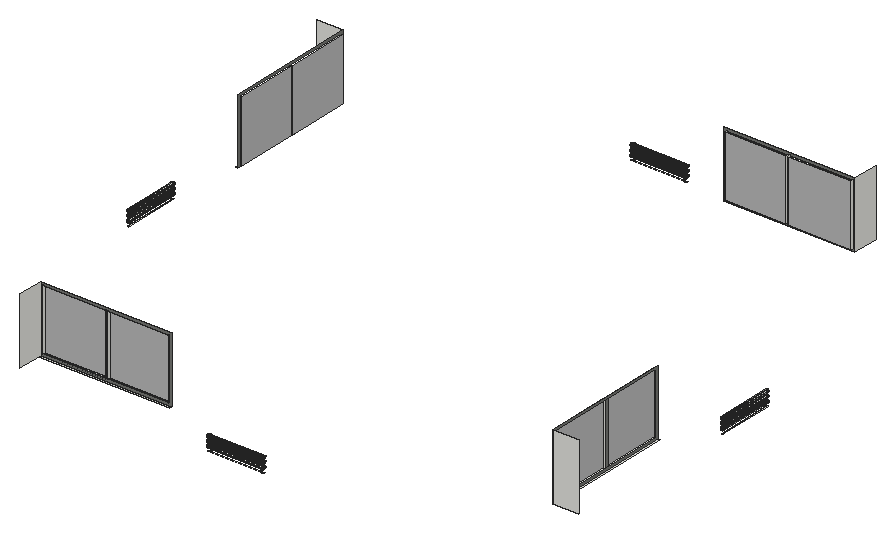
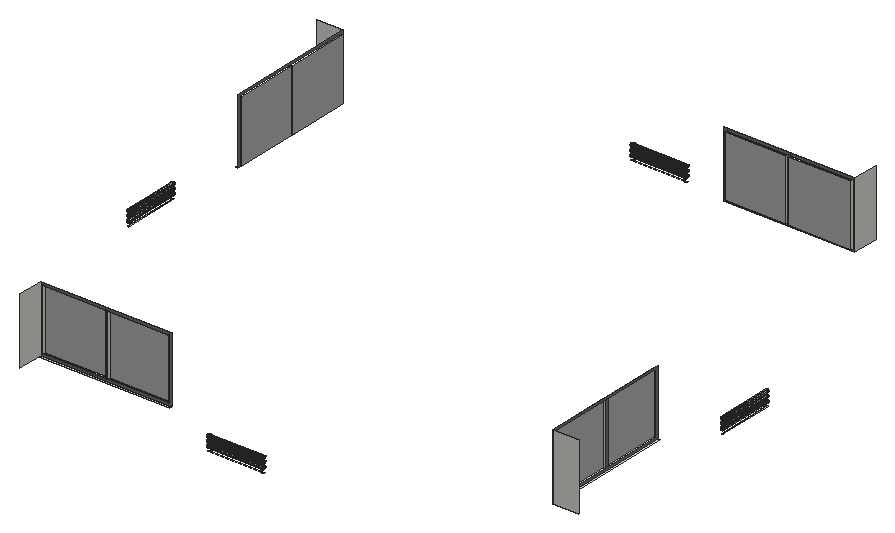
# SketchUp Ruby script. Lengths in inches.
U = 1.inch
M = Sketchup.active_model
def pt(a) = Geom::Point3d.new(a.map { |v| v * U })
def face(e, loops, mat)
  f = e.add_face(loops[0].map { |a| pt(a) })
  loops[1..].each { |l| e.add_face(l.map { |a| pt(a) }).erase! }
  f.material = f.back_material = mat if mat
  f
end
# faces: each face lists its corners as indices into pts; further lists are holes
def faces(e, pts, list, mat = nil) = list.each { |f| face(e, (f[0].is_a?(Array) ? f : [f]).map { |l| l.map { |i| pts[i] } }, mat) }
# xy, xz, yz: faces in a plane at the given z, y or x. An outline is a flat list of corners, or four numbers for a rectangle; further outlines are holes
def ring(l) = l.size == 4 ? [[l[0], l[1]], [l[2], l[1]], [l[2], l[3]], [l[0], l[3]]] : l.each_slice(2).to_a
def flat(e, list, mat, &to3) = list.each { |f| face(e, (f[0].is_a?(Array) ? f : [f]).map { |l| ring(l).map { |u, v| to3.(u, v) } }, mat) }
def xy(e, z, list, mat = nil) = flat(e, list, mat) { |x, y| [x, y, z] }
def xz(e, y, list, mat = nil) = flat(e, list, mat) { |x, z| [x, y, z] }
def yz(e, x, list, mat = nil) = flat(e, list, mat) { |y, z| [x, y, z] }
def lines(e, pts, list) = list.each { |a, b| e.add_line(pt(pts[a]), pt(pts[b])) }
# prism: a flat outline (further loops are holes) pulled along v
def prism(e, loops, v, mat = nil)
  f = face(e, loops, mat); d = Geom::Vector3d.new(v.map { |x| x * U })
  f.pushpull(f.normal.samedirection?(d) ? d.length : -d.length)
end
def box(e, o, s, mat = nil) = prism(e, [[o, [o[0] + s[0], o[1], o[2]], [o[0] + s[0], o[1] + s[1], o[2]], [o[0], o[1] + s[1], o[2]]]], [0, 0, s[2]], mat)
def at(x, y, z, deg = 0) = Geom::Transformation.translation(pt([x, y, z])) * Geom::Transformation.rotation(ORIGIN, Z_AXIS, deg.degrees)
def axes(o, x, y, z) = Geom::Transformation.new([*x, 0, *y, 0, *z, 0, *pt(o).to_a, 1])
def part(name) = M.definitions.add(name)
# library, detail: a bought-in or finely detailed component or shape, given as its bounding box
def library(name, o, s) = part(name).tap { |d| box(d.entities, o, s) }
def detail(e, o, s) = box(e.add_group.entities, o, s)
def put(e, d, t, mat = nil) = e.add_instance(d, t).tap { |i| i.material = mat if mat }
def group(e, t, mat = nil) = e.add_group.tap { |g| g.transformation = t; g.material = mat if mat }.entities
root = M.entities
M.materials.add("[Metal Seamed]").color = [118, 119, 115]
M.materials.add("[Mirror 01]").color = [185, 185, 185]
xy(root,1253.76,[[306.65,96.8125,641.22,102.8125],[1482,271.47,1488,606.03],[132,943.59,138,1278.16],[978.78,1446.8125,1313.35,1452.8125]])
xy(root,1259.76,[[312.65,102.8125,473.9375,108.8125],[479.9375,102.8125,635.22,108.8125],[1476,277.47,1482,438.75],[1476,444.75,1482,600.03],[138,949.59,144,1104.875],
  [138,1110.875,144,1272.16],[984.78,1440.8125,1140.0625,1446.8125],[1146.0625,1440.8125,1307.35,1446.8125]])
xz(root,102.8125,[[[306.65,1253.76,641.22,1422.625],[312.65,1259.76,635.22,1416.625]],[473.9375,1259.76,479.9375,1416.625]],"[Metal Seamed]")
xz(root,108.8125,[[312.65,1259.76,473.9375,1416.625],[479.9375,1259.76,635.22,1416.625]],"[Mirror 01]")
xz(root,271.47,[[1482,1253.76,1548,1422.625]])
xz(root,277.47,[[1476,1259.76,1482,1416.625]])
xz(root,438.75,[[1476,1259.76,1482,1416.625]])
xz(root,444.75,[[1476,1259.76,1482,1416.625]])
xz(root,600.03,[[1476,1259.76,1482,1416.625]])
xz(root,949.59,[[138,1259.76,144,1416.625]])
xz(root,1104.875,[[138,1259.76,144,1416.625]])
xz(root,1110.875,[[138,1259.76,144,1416.625]])
xz(root,1272.16,[[138,1259.76,144,1416.625]])
xz(root,1278.16,[[72,1253.76,138,1422.625]])
xz(root,1440.8125,[[984.78,1259.76,1140.0625,1416.625],[1146.0625,1259.76,1307.35,1416.625]],"[Mirror 01]")
xz(root,1446.8125,[[[978.78,1253.76,1313.35,1422.625],[984.78,1259.76,1307.35,1416.625]],[1140.0625,1259.76,1146.0625,1416.625]],"[Metal Seamed]")
yz(root,138,[[[943.59,1253.76,1278.16,1422.625],[949.59,1259.76,1272.16,1416.625]],[1104.875,1259.76,1110.875,1416.625]],"[Metal Seamed]")
yz(root,144,[[949.59,1259.76,1104.875,1416.625],[1110.875,1259.76,1272.16,1416.625]],"[Mirror 01]")
yz(root,306.65,[[36.8125,1253.76,102.8125,1422.625]])
yz(root,312.65,[[102.8125,1259.76,108.8125,1416.625]])
yz(root,473.9375,[[102.8125,1259.76,108.8125,1416.625]],"[Metal Seamed]")
yz(root,479.9375,[[102.8125,1259.76,108.8125,1416.625]])
yz(root,635.22,[[102.8125,1259.76,108.8125,1416.625]],"[Metal Seamed]")
yz(root,984.78,[[1440.8125,1259.76,1446.8125,1416.625]])
yz(root,1140.0625,[[1440.8125,1259.76,1446.8125,1416.625]])
yz(root,1146.0625,[[1440.8125,1259.76,1446.8125,1416.625]])
yz(root,1307.35,[[1440.8125,1259.76,1446.8125,1416.625]])
yz(root,1313.35,[[1446.8125,1253.76,1512.8125,1422.625]])
yz(root,1476,[[277.47,1259.76,438.75,1416.625],[444.75,1259.76,600.03,1416.625]],"[Mirror 01]")
yz(root,1482,[[[271.47,1253.76,606.03,1422.625],[277.47,1259.76,600.03,1416.625]],[438.75,1259.76,444.75,1416.625]],"[Metal Seamed]")
p = [[922.01,46.5,1224.9],[922.01,47.38,1225.27],[778.64,47.38,1225.27],[778.64,46.5,1224.9],[922.01,49.29,1225.27],[922.01,50.18,1224.9],
  [778.64,50.18,1224.9],[778.64,49.29,1225.27],[81.68,662.8,1224.9],[82.57,662.8,1225.27],[82.57,806.17,1225.27],[81.68,806.17,1224.9],
  [84.48,662.8,1225.27],[85.37,662.8,1224.9],[85.37,806.17,1224.9],[84.48,806.17,1225.27],[1535.52,886.83,1225.27],[1534.63,886.83,1224.9],
  [1534.63,743.45,1224.9],[1535.52,743.45,1225.27],[1538.32,886.83,1224.9],[1537.43,886.83,1225.27],[1537.43,743.45,1225.27],[1538.32,743.45,1224.9],
  [697.99,1500.33,1225.27],[697.99,1499.44,1224.9],[841.36,1499.44,1224.9],[841.36,1500.33,1225.27],[697.99,1503.13,1224.9],[697.99,1502.24,1225.27],
  [841.36,1502.24,1225.27],[841.36,1503.13,1224.9],[922.01,48.34,1225.39],[778.64,48.34,1225.39],[83.53,662.8,1225.39],[83.53,806.17,1225.39],
  [1536.47,886.83,1225.39],[1536.47,743.45,1225.39],[697.99,1501.28,1225.39],[841.36,1501.28,1225.39],[922.01,48.34,1233.02],[922.01,47.38,1233.14],
  [778.64,47.38,1233.14],[778.64,48.34,1233.02],[922.01,49.29,1233.14],[778.64,49.29,1233.14],[83.53,662.8,1233.02],[82.57,662.8,1233.14],
  [82.57,806.17,1233.14],[83.53,806.17,1233.02],[84.48,662.8,1233.14],[84.48,806.17,1233.14],[1535.52,886.83,1233.14],[1536.47,886.83,1233.02],
  [1536.47,743.45,1233.02],[1535.52,743.45,1233.14],[1537.43,886.83,1233.14],[1537.43,743.45,1233.14],[697.99,1500.33,1233.14],[697.99,1501.28,1233.02],
  [841.36,1501.28,1233.02],[841.36,1500.33,1233.14],[697.99,1502.24,1233.14],[841.36,1502.24,1233.14],[922.01,46.5,1233.51],[778.64,46.5,1233.51],
  [922.01,50.18,1233.51],[778.64,50.18,1233.51],[81.68,662.8,1233.51],[81.68,806.17,1233.51],[85.37,662.8,1233.51],[85.37,806.17,1233.51],
  [1534.63,886.83,1233.51],[1534.63,743.45,1233.51],[1538.32,886.83,1233.51],[1538.32,743.45,1233.51],[697.99,1499.44,1233.51],[841.36,1499.44,1233.51],
  [697.99,1503.13,1233.51],[841.36,1503.13,1233.51],[922.01,45.73,1234.1],[778.64,45.73,1234.1],[922.01,50.95,1234.1],[778.64,50.95,1234.1],
  [80.92,662.8,1234.1],[80.92,806.17,1234.1],[86.13,662.8,1234.1],[86.13,806.17,1234.1],[1533.87,886.83,1234.1],[1533.87,743.45,1234.1],
  [1539.08,886.83,1234.1],[1539.08,743.45,1234.1],[697.99,1498.68,1234.1],[841.36,1498.68,1234.1],[697.99,1503.89,1234.1],[841.36,1503.89,1234.1],
  [922.01,45.15,1234.86],[778.64,45.15,1234.86],[922.01,51.53,1234.86],[778.64,51.53,1234.86],[80.33,662.8,1234.86],[80.33,806.17,1234.86],
  [86.72,662.8,1234.86],[86.72,806.17,1234.86],[1533.28,886.83,1234.86],[1533.28,743.45,1234.86],[1539.67,886.83,1234.86],[1539.67,743.45,1234.86],
  [697.99,1498.09,1234.86],[841.36,1498.09,1234.86],[697.99,1504.48,1234.86],[841.36,1504.48,1234.86],[922.01,44.78,1235.75],[778.64,44.78,1235.75],
  [922.01,51.9,1235.75],[778.64,51.9,1235.75],[79.97,662.8,1235.75],[79.97,806.17,1235.75],[87.09,662.8,1235.75],[87.09,806.17,1235.75],
  [1532.91,886.83,1235.75],[1532.91,743.45,1235.75],[1540.03,886.83,1235.75],[1540.03,743.45,1235.75],[697.99,1497.72,1235.75],[841.36,1497.72,1235.75],
  [697.99,1504.85,1235.75],[841.36,1504.85,1235.75],[922.01,44.65,1236.7],[778.64,44.65,1236.7],[922.01,52.03,1236.7],[778.64,52.03,1236.7],
  [79.84,662.8,1236.7],[79.84,806.17,1236.7],[87.21,662.8,1236.7],[87.21,806.17,1236.7],[1532.79,886.83,1236.7],[1532.79,743.45,1236.7],
  [1540.16,886.83,1236.7],[1540.16,743.45,1236.7],[697.99,1497.6,1236.7],[841.36,1497.6,1236.7],[697.99,1504.97,1236.7],[841.36,1504.97,1236.7],
  [922.01,44.78,1237.66],[778.64,44.78,1237.66],[922.01,51.9,1237.66],[778.64,51.9,1237.66],[79.97,662.8,1237.66],[79.97,806.17,1237.66],
  [87.09,662.8,1237.66],[87.09,806.17,1237.66],[1532.91,886.83,1237.66],[1532.91,743.45,1237.66],[1540.03,886.83,1237.66],[1540.03,743.45,1237.66],
  [697.99,1497.72,1237.66],[841.36,1497.72,1237.66],[697.99,1504.85,1237.66],[841.36,1504.85,1237.66],[922.01,45.15,1238.55],[778.64,45.15,1238.55],
  [922.01,51.53,1238.55],[778.64,51.53,1238.55],[80.33,662.8,1238.55],[80.33,806.17,1238.55],[86.72,662.8,1238.55],[86.72,806.17,1238.55],
  [1533.28,886.83,1238.55],[1533.28,743.45,1238.55],[1539.67,886.83,1238.55],[1539.67,743.45,1238.55],[697.99,1498.09,1238.55],[841.36,1498.09,1238.55],
  [697.99,1504.48,1238.55],[841.36,1504.48,1238.55],[922.01,45.73,1239.3125],[778.64,45.73,1239.3125],[922.01,50.95,1239.3125],[778.64,50.95,1239.3125],
  [80.92,662.8,1239.3125],[80.92,806.17,1239.3125],[86.13,662.8,1239.3125],[86.13,806.17,1239.3125],[1533.87,886.83,1239.3125],[1533.87,743.45,1239.3125],
  [1539.08,886.83,1239.3125],[1539.08,743.45,1239.3125],[697.99,1498.68,1239.3125],[841.36,1498.68,1239.3125],[697.99,1503.89,1239.3125],[841.36,1503.89,1239.3125],
  [922.01,46.5,1239.9],[778.64,46.5,1239.9],[922.01,50.18,1239.9],[778.64,50.18,1239.9],[81.68,662.8,1239.9],[81.68,806.17,1239.9],
  [85.37,662.8,1239.9],[85.37,806.17,1239.9],[1534.63,886.83,1239.9],[1534.63,743.45,1239.9],[1538.32,886.83,1239.9],[1538.32,743.45,1239.9],
  [697.99,1499.44,1239.9],[841.36,1499.44,1239.9],[697.99,1503.13,1239.9],[841.36,1503.13,1239.9],[922.01,47.38,1240.27],[778.64,47.38,1240.27],
  [922.01,49.29,1240.27],[778.64,49.29,1240.27],[82.57,662.8,1240.27],[82.57,806.17,1240.27],[84.48,662.8,1240.27],[84.48,806.17,1240.27],
  [1535.52,886.83,1240.27],[1535.52,743.45,1240.27],[1537.43,886.83,1240.27],[1537.43,743.45,1240.27],[697.99,1500.33,1240.27],[841.36,1500.33,1240.27],
  [697.99,1502.24,1240.27],[841.36,1502.24,1240.27],[922.01,48.34,1240.39],[778.64,48.34,1240.39],[83.53,662.8,1240.39],[83.53,806.17,1240.39],
  [1536.47,886.83,1240.39],[1536.47,743.45,1240.39],[697.99,1501.28,1240.39],[841.36,1501.28,1240.39],[922.01,48.34,1245.02],[922.01,47.38,1245.14],
  [778.64,47.38,1245.14],[778.64,48.34,1245.02],[922.01,49.29,1245.14],[778.64,49.29,1245.14],[83.53,662.8,1245.02],[82.57,662.8,1245.14],
  [82.57,806.17,1245.14],[83.53,806.17,1245.02],[84.48,662.8,1245.14],[84.48,806.17,1245.14],[1535.52,886.83,1245.14],[1536.47,886.83,1245.02],
  [1536.47,743.45,1245.02],[1535.52,743.45,1245.14],[1537.43,886.83,1245.14],[1537.43,743.45,1245.14],[697.99,1500.33,1245.14],[697.99,1501.28,1245.02],
  [841.36,1501.28,1245.02],[841.36,1500.33,1245.14],[697.99,1502.24,1245.14],[841.36,1502.24,1245.14],[922.01,46.5,1245.51],[778.64,46.5,1245.51],
  [922.01,50.18,1245.51],[778.64,50.18,1245.51],[81.68,662.8,1245.51],[81.68,806.17,1245.51],[85.37,662.8,1245.51],[85.37,806.17,1245.51],
  [1534.63,886.83,1245.51],[1534.63,743.45,1245.51],[1538.32,886.83,1245.51],[1538.32,743.45,1245.51],[697.99,1499.44,1245.51],[841.36,1499.44,1245.51],
  [697.99,1503.13,1245.51],[841.36,1503.13,1245.51],[922.01,45.73,1246.1],[778.64,45.73,1246.1],[922.01,50.95,1246.1],[778.64,50.95,1246.1],
  [80.92,662.8,1246.1],[80.92,806.17,1246.1],[86.13,662.8,1246.1],[86.13,806.17,1246.1],[1533.87,886.83,1246.1],[1533.87,743.45,1246.1],
  [1539.08,886.83,1246.1],[1539.08,743.45,1246.1],[697.99,1498.68,1246.1],[841.36,1498.68,1246.1],[697.99,1503.89,1246.1],[841.36,1503.89,1246.1],
  [922.01,45.15,1246.86],[778.64,45.15,1246.86],[922.01,51.53,1246.86],[778.64,51.53,1246.86],[80.33,662.8,1246.86],[80.33,806.17,1246.86],
  [86.72,662.8,1246.86],[86.72,806.17,1246.86],[1533.28,886.83,1246.86],[1533.28,743.45,1246.86],[1539.67,886.83,1246.86],[1539.67,743.45,1246.86],
  [697.99,1498.09,1246.86],[841.36,1498.09,1246.86],[697.99,1504.48,1246.86],[841.36,1504.48,1246.86],[922.01,44.78,1247.75],[778.64,44.78,1247.75],
  [922.01,51.9,1247.75],[778.64,51.9,1247.75],[79.97,662.8,1247.75],[79.97,806.17,1247.75],[87.09,662.8,1247.75],[87.09,806.17,1247.75],
  [1532.91,886.83,1247.75],[1532.91,743.45,1247.75],[1540.03,886.83,1247.75],[1540.03,743.45,1247.75],[697.99,1497.72,1247.75],[841.36,1497.72,1247.75],
  [697.99,1504.85,1247.75],[841.36,1504.85,1247.75],[922.01,44.65,1248.7],[778.64,44.65,1248.7],[922.01,52.03,1248.7],[778.64,52.03,1248.7],
  [79.84,662.8,1248.7],[79.84,806.17,1248.7],[87.21,662.8,1248.7],[87.21,806.17,1248.7],[1532.79,886.83,1248.7],[1532.79,743.45,1248.7],
  [1540.16,886.83,1248.7],[1540.16,743.45,1248.7],[697.99,1497.6,1248.7],[841.36,1497.6,1248.7],[697.99,1504.97,1248.7],[841.36,1504.97,1248.7],
  [922.01,44.78,1249.66],[778.64,44.78,1249.66],[922.01,51.9,1249.66],[778.64,51.9,1249.66],[79.97,662.8,1249.66],[79.97,806.17,1249.66],
  [87.09,662.8,1249.66],[87.09,806.17,1249.66],[1532.91,886.83,1249.66],[1532.91,743.45,1249.66],[1540.03,886.83,1249.66],[1540.03,743.45,1249.66],
  [697.99,1497.72,1249.66],[841.36,1497.72,1249.66],[697.99,1504.85,1249.66],[841.36,1504.85,1249.66],[922.01,45.15,1250.55],[778.64,45.15,1250.55],
  [922.01,51.53,1250.55],[778.64,51.53,1250.55],[80.33,662.8,1250.55],[80.33,806.17,1250.55],[86.72,662.8,1250.55],[86.72,806.17,1250.55],
  [1533.28,886.83,1250.55],[1533.28,743.45,1250.55],[1539.67,886.83,1250.55],[1539.67,743.45,1250.55],[697.99,1498.09,1250.55],[841.36,1498.09,1250.55],
  [697.99,1504.48,1250.55],[841.36,1504.48,1250.55],[922.01,45.73,1251.3125],[778.64,45.73,1251.3125],[922.01,50.95,1251.3125],[778.64,50.95,1251.3125],
  [80.92,662.8,1251.3125],[80.92,806.17,1251.3125],[86.13,662.8,1251.3125],[86.13,806.17,1251.3125],[1533.87,886.83,1251.3125],[1533.87,743.45,1251.3125],
  [1539.08,886.83,1251.3125],[1539.08,743.45,1251.3125],[697.99,1498.68,1251.3125],[841.36,1498.68,1251.3125],[697.99,1503.89,1251.3125],[841.36,1503.89,1251.3125],
  [922.01,46.5,1251.9],[778.64,46.5,1251.9],[922.01,50.18,1251.9],[778.64,50.18,1251.9],[81.68,662.8,1251.9],[81.68,806.17,1251.9],
  [85.37,662.8,1251.9],[85.37,806.17,1251.9],[1534.63,886.83,1251.9],[1534.63,743.45,1251.9],[1538.32,886.83,1251.9],[1538.32,743.45,1251.9],
  [697.99,1499.44,1251.9],[841.36,1499.44,1251.9],[697.99,1503.13,1251.9],[841.36,1503.13,1251.9],[922.01,47.38,1252.27],[778.64,47.38,1252.27],
  [922.01,49.29,1252.27],[778.64,49.29,1252.27],[82.57,662.8,1252.27],[82.57,806.17,1252.27],[84.48,662.8,1252.27],[84.48,806.17,1252.27],
  [1535.52,886.83,1252.27],[1535.52,743.45,1252.27],[1537.43,886.83,1252.27],[1537.43,743.45,1252.27],[697.99,1500.33,1252.27],[841.36,1500.33,1252.27],
  [697.99,1502.24,1252.27],[841.36,1502.24,1252.27],[922.01,48.34,1252.39],[778.64,48.34,1252.39],[83.53,662.8,1252.39],[83.53,806.17,1252.39],
  [1536.47,886.83,1252.39],[1536.47,743.45,1252.39],[697.99,1501.28,1252.39],[841.36,1501.28,1252.39],[922.01,48.34,1257.02],[922.01,47.38,1257.14],
  [778.64,47.38,1257.14],[778.64,48.34,1257.02],[922.01,49.29,1257.14],[778.64,49.29,1257.14],[83.53,662.8,1257.02],[82.57,662.8,1257.14],
  [82.57,806.17,1257.14],[83.53,806.17,1257.02],[84.48,662.8,1257.14],[84.48,806.17,1257.14],[1535.52,886.83,1257.14],[1536.47,886.83,1257.02],
  [1536.47,743.45,1257.02],[1535.52,743.45,1257.14],[1537.43,886.83,1257.14],[1537.43,743.45,1257.14],[697.99,1500.33,1257.14],[697.99,1501.28,1257.02],
  [841.36,1501.28,1257.02],[841.36,1500.33,1257.14],[697.99,1502.24,1257.14],[841.36,1502.24,1257.14],[922.01,46.5,1257.51],[778.64,46.5,1257.51],
  [922.01,50.18,1257.51],[778.64,50.18,1257.51],[81.68,662.8,1257.51],[81.68,806.17,1257.51],[85.37,662.8,1257.51],[85.37,806.17,1257.51],
  [1534.63,886.83,1257.51],[1534.63,743.45,1257.51],[1538.32,886.83,1257.51],[1538.32,743.45,1257.51],[697.99,1499.44,1257.51],[841.36,1499.44,1257.51],
  [697.99,1503.13,1257.51],[841.36,1503.13,1257.51],[922.01,45.73,1258.1],[778.64,45.73,1258.1],[922.01,50.95,1258.1],[778.64,50.95,1258.1],
  [80.92,662.8,1258.1],[80.92,806.17,1258.1],[86.13,662.8,1258.1],[86.13,806.17,1258.1],[1533.87,886.83,1258.1],[1533.87,743.45,1258.1],
  [1539.08,886.83,1258.1],[1539.08,743.45,1258.1],[697.99,1498.68,1258.1],[841.36,1498.68,1258.1],[697.99,1503.89,1258.1],[841.36,1503.89,1258.1],
  [922.01,45.15,1258.86],[778.64,45.15,1258.86],[922.01,51.53,1258.86],[778.64,51.53,1258.86],[80.33,662.8,1258.86],[80.33,806.17,1258.86],
  [86.72,662.8,1258.86],[86.72,806.17,1258.86],[1533.28,886.83,1258.86],[1533.28,743.45,1258.86],[1539.67,886.83,1258.86],[1539.67,743.45,1258.86],
  [697.99,1498.09,1258.86],[841.36,1498.09,1258.86],[697.99,1504.48,1258.86],[841.36,1504.48,1258.86],[922.01,44.78,1259.75],[778.64,44.78,1259.75],
  [922.01,51.9,1259.75],[778.64,51.9,1259.75],[79.97,662.8,1259.75],[79.97,806.17,1259.75],[87.09,662.8,1259.75],[87.09,806.17,1259.75],
  [1532.91,886.83,1259.75],[1532.91,743.45,1259.75],[1540.03,886.83,1259.75],[1540.03,743.45,1259.75],[697.99,1497.72,1259.75],[841.36,1497.72,1259.75],
  [697.99,1504.85,1259.75],[841.36,1504.85,1259.75],[922.01,44.65,1260.7],[778.64,44.65,1260.7],[922.01,52.03,1260.7],[778.64,52.03,1260.7],
  [79.84,662.8,1260.7],[79.84,806.17,1260.7],[87.21,662.8,1260.7],[87.21,806.17,1260.7],[1532.79,886.83,1260.7],[1532.79,743.45,1260.7],
  [1540.16,886.83,1260.7],[1540.16,743.45,1260.7],[697.99,1497.6,1260.7],[841.36,1497.6,1260.7],[697.99,1504.97,1260.7],[841.36,1504.97,1260.7],
  [922.01,44.78,1261.66],[778.64,44.78,1261.66],[922.01,51.9,1261.66],[778.64,51.9,1261.66],[79.97,662.8,1261.66],[79.97,806.17,1261.66],
  [87.09,662.8,1261.66],[87.09,806.17,1261.66],[1532.91,886.83,1261.66],[1532.91,743.45,1261.66],[1540.03,886.83,1261.66],[1540.03,743.45,1261.66],
  [697.99,1497.72,1261.66],[841.36,1497.72,1261.66],[697.99,1504.85,1261.66],[841.36,1504.85,1261.66],[922.01,45.15,1262.55],[778.64,45.15,1262.55],
  [922.01,51.53,1262.55],[778.64,51.53,1262.55],[80.33,662.8,1262.55],[80.33,806.17,1262.55],[86.72,662.8,1262.55],[86.72,806.17,1262.55],
  [1533.28,886.83,1262.55],[1533.28,743.45,1262.55],[1539.67,886.83,1262.55],[1539.67,743.45,1262.55],[697.99,1498.09,1262.55],[841.36,1498.09,1262.55],
  [697.99,1504.48,1262.55],[841.36,1504.48,1262.55],[922.01,45.73,1263.3125],[778.64,45.73,1263.3125],[922.01,50.95,1263.3125],[778.64,50.95,1263.3125],
  [80.92,662.8,1263.3125],[80.92,806.17,1263.3125],[86.13,662.8,1263.3125],[86.13,806.17,1263.3125],[1533.87,886.83,1263.3125],[1533.87,743.45,1263.3125],
  [1539.08,886.83,1263.3125],[1539.08,743.45,1263.3125],[697.99,1498.68,1263.3125],[841.36,1498.68,1263.3125],[697.99,1503.89,1263.3125],[841.36,1503.89,1263.3125],
  [922.01,46.5,1263.9],[778.64,46.5,1263.9],[922.01,50.18,1263.9],[778.64,50.18,1263.9],[81.68,662.8,1263.9],[81.68,806.17,1263.9],
  [85.37,662.8,1263.9],[85.37,806.17,1263.9],[1534.63,886.83,1263.9],[1534.63,743.45,1263.9],[1538.32,886.83,1263.9],[1538.32,743.45,1263.9],
  [697.99,1499.44,1263.9],[841.36,1499.44,1263.9],[697.99,1503.13,1263.9],[841.36,1503.13,1263.9],[922.01,47.38,1264.27],[778.64,47.38,1264.27],
  [922.01,49.29,1264.27],[778.64,49.29,1264.27],[82.57,662.8,1264.27],[82.57,806.17,1264.27],[84.48,662.8,1264.27],[84.48,806.17,1264.27],
  [1535.52,886.83,1264.27],[1535.52,743.45,1264.27],[1537.43,886.83,1264.27],[1537.43,743.45,1264.27],[697.99,1500.33,1264.27],[841.36,1500.33,1264.27],
  [697.99,1502.24,1264.27],[841.36,1502.24,1264.27],[922.01,48.34,1264.39],[778.64,48.34,1264.39],[83.53,662.8,1264.39],[83.53,806.17,1264.39],
  [1536.47,886.83,1264.39],[1536.47,743.45,1264.39],[697.99,1501.28,1264.39],[841.36,1501.28,1264.39]]
faces(root,p,[[0,1,2,3],[4,5,6,7],[8,9,10,11],[12,13,14,15],[16,17,18,19],[20,21,22,23],[24,25,26,27],[28,29,30,31],
  [1,32,33,2],[32,4,7,33],[9,34,35,10],[34,12,15,35],[36,16,19,37],[21,36,37,22],[38,24,27,39],[29,38,39,30],
  [40,41,42,43],[44,40,43,45],[46,47,48,49],[50,46,49,51],[52,53,54,55],[53,56,57,54],[58,59,60,61],[59,62,63,60],
  [41,64,65,42],[66,44,45,67],[47,68,69,48],[70,50,51,71],[72,52,55,73],[56,74,75,57],[76,58,61,77],[62,78,79,63],
  [64,80,81,65],[82,66,67,83],[68,84,85,69],[86,70,71,87],[88,72,73,89],[74,90,91,75],[92,76,77,93],[78,94,95,79],
  [80,96,97,81],[98,82,83,99],[84,100,101,85],[102,86,87,103],[104,88,89,105],[90,106,107,91],[108,92,93,109],[94,110,111,95],
  [96,112,113,97],[114,98,99,115],[100,116,117,101],[118,102,103,119],[120,104,105,121],[106,122,123,107],[124,108,109,125],[110,126,127,111],
  [112,128,129,113],[130,114,115,131],[116,132,133,117],[134,118,119,135],[136,120,121,137],[122,138,139,123],[140,124,125,141],[126,142,143,127],
  [128,144,145,129],[146,130,131,147],[132,148,149,133],[150,134,135,151],[152,136,137,153],[138,154,155,139],[156,140,141,157],[142,158,159,143],
  [144,160,161,145],[162,146,147,163],[148,164,165,149],[166,150,151,167],[168,152,153,169],[154,170,171,155],[172,156,157,173],[158,174,175,159],
  [160,176,177,161],[178,162,163,179],[164,180,181,165],[182,166,167,183],[184,168,169,185],[170,186,187,171],[188,172,173,189],[174,190,191,175],
  [176,192,193,177],[194,178,179,195],[180,196,197,181],[198,182,183,199],[200,184,185,201],[186,202,203,187],[204,188,189,205],[190,206,207,191],
  [192,208,209,193],[210,194,195,211],[196,212,213,197],[214,198,199,215],[216,200,201,217],[202,218,219,203],[220,204,205,221],[206,222,223,207],
  [208,224,225,209],[224,210,211,225],[212,226,227,213],[226,214,215,227],[228,216,217,229],[218,228,229,219],[230,220,221,231],[222,230,231,223],
  [232,233,234,235],[236,232,235,237],[238,239,240,241],[242,238,241,243],[244,245,246,247],[245,248,249,246],[250,251,252,253],[251,254,255,252],
  [233,256,257,234],[258,236,237,259],[239,260,261,240],[262,242,243,263],[264,244,247,265],[248,266,267,249],[268,250,253,269],[254,270,271,255],
  [256,272,273,257],[274,258,259,275],[260,276,277,261],[278,262,263,279],[280,264,265,281],[266,282,283,267],[284,268,269,285],[270,286,287,271],
  [272,288,289,273],[290,274,275,291],[276,292,293,277],[294,278,279,295],[296,280,281,297],[282,298,299,283],[300,284,285,301],[286,302,303,287],
  [288,304,305,289],[306,290,291,307],[292,308,309,293],[310,294,295,311],[312,296,297,313],[298,314,315,299],[316,300,301,317],[302,318,319,303],
  [304,320,321,305],[322,306,307,323],[308,324,325,309],[326,310,311,327],[328,312,313,329],[314,330,331,315],[332,316,317,333],[318,334,335,319],
  [320,336,337,321],[338,322,323,339],[324,340,341,325],[342,326,327,343],[344,328,329,345],[330,346,347,331],[348,332,333,349],[334,350,351,335],
  [336,352,353,337],[354,338,339,355],[340,356,357,341],[358,342,343,359],[360,344,345,361],[346,362,363,347],[364,348,349,365],[350,366,367,351],
  [352,368,369,353],[370,354,355,371],[356,372,373,357],[374,358,359,375],[376,360,361,377],[362,378,379,363],[380,364,365,381],[366,382,383,367],
  [368,384,385,369],[386,370,371,387],[372,388,389,373],[390,374,375,391],[392,376,377,393],[378,394,395,379],[396,380,381,397],[382,398,399,383],
  [384,400,401,385],[402,386,387,403],[388,404,405,389],[406,390,391,407],[408,392,393,409],[394,410,411,395],[412,396,397,413],[398,414,415,399],
  [400,416,417,401],[416,402,403,417],[404,418,419,405],[418,406,407,419],[420,408,409,421],[410,420,421,411],[422,412,413,423],[414,422,423,415],
  [424,425,426,427],[428,424,427,429],[430,431,432,433],[434,430,433,435],[436,437,438,439],[437,440,441,438],[442,443,444,445],[443,446,447,444],
  [425,448,449,426],[450,428,429,451],[431,452,453,432],[454,434,435,455],[456,436,439,457],[440,458,459,441],[460,442,445,461],[446,462,463,447],
  [448,464,465,449],[466,450,451,467],[452,468,469,453],[470,454,455,471],[472,456,457,473],[458,474,475,459],[476,460,461,477],[462,478,479,463],
  [464,480,481,465],[482,466,467,483],[468,484,485,469],[486,470,471,487],[488,472,473,489],[474,490,491,475],[492,476,477,493],[478,494,495,479],
  [480,496,497,481],[498,482,483,499],[484,500,501,485],[502,486,487,503],[504,488,489,505],[490,506,507,491],[508,492,493,509],[494,510,511,495],
  [496,512,513,497],[514,498,499,515],[500,516,517,501],[518,502,503,519],[520,504,505,521],[506,522,523,507],[524,508,509,525],[510,526,527,511],
  [512,528,529,513],[530,514,515,531],[516,532,533,517],[534,518,519,535],[536,520,521,537],[522,538,539,523],[540,524,525,541],[526,542,543,527],
  [528,544,545,529],[546,530,531,547],[532,548,549,533],[550,534,535,551],[552,536,537,553],[538,554,555,539],[556,540,541,557],[542,558,559,543],
  [544,560,561,545],[562,546,547,563],[548,564,565,549],[566,550,551,567],[568,552,553,569],[554,570,571,555],[572,556,557,573],[558,574,575,559],
  [560,576,577,561],[578,562,563,579],[564,580,581,565],[582,566,567,583],[584,568,569,585],[570,586,587,571],[588,572,573,589],[574,590,591,575],
  [576,592,593,577],[594,578,579,595],[580,596,597,581],[598,582,583,599],[600,584,585,601],[586,602,603,587],[604,588,589,605],[590,606,607,591],
  [592,608,609,593],[608,594,595,609],[596,610,611,597],[610,598,599,611],[612,600,601,613],[602,612,613,603],[614,604,605,615],[606,614,615,607]])
